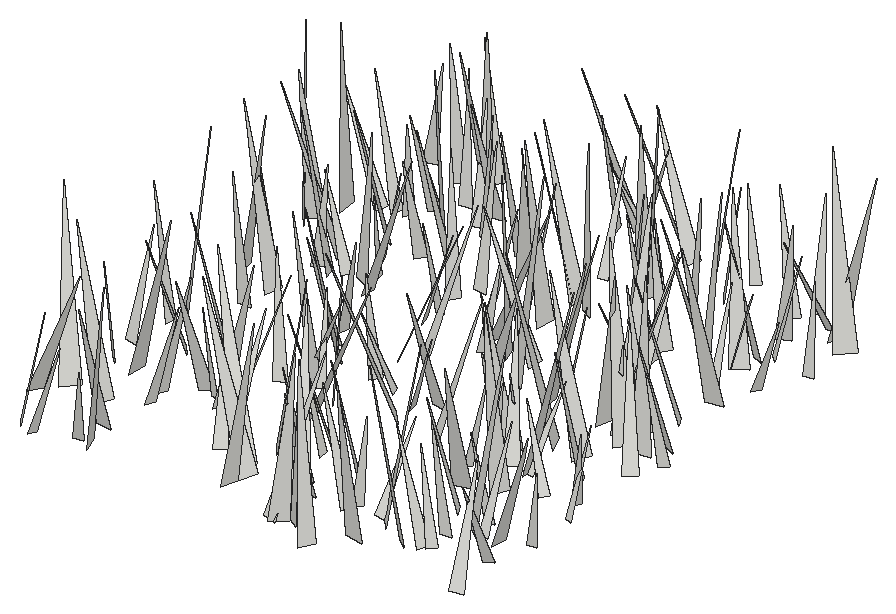
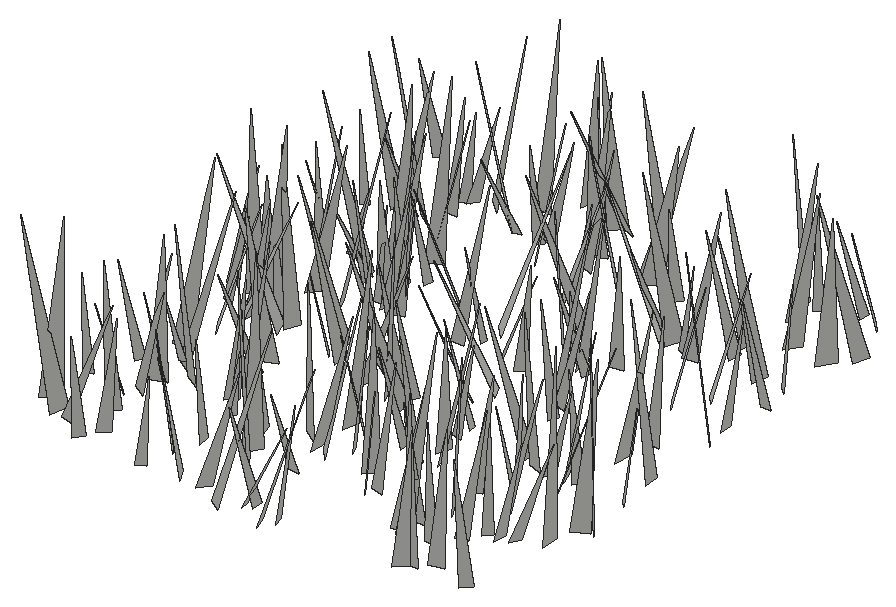
# SketchUp Ruby script. Lengths in inches.
U = 1.inch
M = Sketchup.active_model
def pt(a) = Geom::Point3d.new(a.map { |v| v * U })
def face(e, loops, mat)
  f = e.add_face(loops[0].map { |a| pt(a) })
  loops[1..].each { |l| e.add_face(l.map { |a| pt(a) }).erase! }
  f.material = f.back_material = mat if mat
  f
end
# faces: each face lists its corners as indices into pts; further lists are holes
def faces(e, pts, list, mat = nil) = list.each { |f| face(e, (f[0].is_a?(Array) ? f : [f]).map { |l| l.map { |i| pts[i] } }, mat) }
# xy, xz, yz: faces in a plane at the given z, y or x. An outline is a flat list of corners, or four numbers for a rectangle; further outlines are holes
def ring(l) = l.size == 4 ? [[l[0], l[1]], [l[2], l[1]], [l[2], l[3]], [l[0], l[3]]] : l.each_slice(2).to_a
def flat(e, list, mat, &to3) = list.each { |f| face(e, (f[0].is_a?(Array) ? f : [f]).map { |l| ring(l).map { |u, v| to3.(u, v) } }, mat) }
def xy(e, z, list, mat = nil) = flat(e, list, mat) { |x, y| [x, y, z] }
def xz(e, y, list, mat = nil) = flat(e, list, mat) { |x, z| [x, y, z] }
def yz(e, x, list, mat = nil) = flat(e, list, mat) { |y, z| [x, y, z] }
def lines(e, pts, list) = list.each { |a, b| e.add_line(pt(pts[a]), pt(pts[b])) }
# prism: a flat outline (further loops are holes) pulled along v
def prism(e, loops, v, mat = nil)
  f = face(e, loops, mat); d = Geom::Vector3d.new(v.map { |x| x * U })
  f.pushpull(f.normal.samedirection?(d) ? d.length : -d.length)
end
def box(e, o, s, mat = nil) = prism(e, [[o, [o[0] + s[0], o[1], o[2]], [o[0] + s[0], o[1] + s[1], o[2]], [o[0], o[1] + s[1], o[2]]]], [0, 0, s[2]], mat)
def at(x, y, z, deg = 0) = Geom::Transformation.translation(pt([x, y, z])) * Geom::Transformation.rotation(ORIGIN, Z_AXIS, deg.degrees)
def axes(o, x, y, z) = Geom::Transformation.new([*x, 0, *y, 0, *z, 0, *pt(o).to_a, 1])
def part(name) = M.definitions.add(name)
# library, detail: a bought-in or finely detailed component or shape, given as its bounding box
def library(name, o, s) = part(name).tap { |d| box(d.entities, o, s) }
def detail(e, o, s) = box(e.add_group.entities, o, s)
def put(e, d, t, mat = nil) = e.add_instance(d, t).tap { |i| i.material = mat if mat }
def group(e, t, mat = nil) = e.add_group.tap { |g| g.transformation = t; g.material = mat if mat }.entities
root = M.entities
c1 = part("fur_instance\#9")
p = [[0.8125,0,1.79],[0.67,-0.02,1.48],[0,-0.11,0],[0,0.11,0]]
faces(c1.entities,p,[[0,1,2,3]])
put(root,c1,axes([454.47,144.27,-21.66],[-5.7343,-4.84539,3.53032],[-5.45543,6.24306,-0.29262],[2.4858,2.5238,7.50162]))
put(root,c1,axes([456.54,114.57,-21.66],[-6.24341,4.5177,1.05822],[4.50521,6.32678,-0.4296],[1.11019,-0.26807,7.69449]))
put(root,c1,axes([456.32,126.54,-21.66],[-5.31115,0.249,1.00047],[0.14264,5.37711,-0.58108],[1.02108,0.54405,5.28514]))
put(root,c1,axes([455.14,139.93,-21.66],[-2.6203,-2.567,1.06702],[-2.53846,2.80716,0.51965],[1.13325,0.35259,3.63117]))
put(root,c1,axes([455.01,145.13,-21.66],[3.62749,-5.55241,1.8821],[-5.65778,-3.89547,-0.58748],[-1.5366,1.23544,6.60627]))
put(root,c1,axes([455.76,147.71,-21.66],[7.3985,0.06507,3.2704],[0.28828,-8.06925,-0.49163],[-3.25831,-0.56619,7.38244]))
put(root,c1,axes([457.83,149.07,-21.66],[-4.93751,1.50851,0.32737],[1.53378,4.91815,0.47027],[0.1741,-0.54591,5.14135]))
put(root,c1,axes([455.94,122.39,-21.66],[0.58745,4.61701,1.14714],[4.75417,-0.52722,-0.31264],[0.17496,-1.17604,4.64372]))
put(root,c1,axes([456.65,119.57,-21.66],[-2.76326,-3.0585,1.38467],[-3.15346,2.97986,0.28892],[1.15213,0.82059,4.11176]))
put(root,c1,axes([455.68,136.01,-21.66],[6.8953,0.9557,1.85973],[1.13553,-7.09282,-0.56526],[-1.75571,-0.83402,6.93822]))
put(root,c1,axes([456.08,128.73,-21.66],[5.70767,4.90783,2.44546],[5.23724,-5.92496,-0.33273],[-1.62433,-1.85811,7.52021]))
put(root,c1,axes([459,149.46,-21.66],[-5.26641,1.25593,0.32091],[1.22212,5.2582,-0.5227],[0.43216,0.43524,5.3888]))
put(root,c1,axes([456.43,156.58,-21.66],[2.66304,-4.00114,1.09323],[-4.14622,-2.60379,0.57024],[-0.11461,1.22768,4.77239]))
put(root,c1,axes([454.9375,112.5,-21.66],[5.86888,-2.59714,0.14419],[-2.59865,-5.83866,0.60558],[0.11385,0.61201,6.38922]))
put(root,c1,axes([459.375,134.63,-21.66],[-7.31689,1.04904,1.18508],[0.99417,7.40794,-0.41938],[1.23147,0.25252,7.3798]))
put(root,c1,axes([459.79,141.79,-21.66],[-6.57116,-2.81105,0.67584],[-2.85659,6.57143,-0.44162],[0.44572,0.67315,7.13352]))
put(root,c1,axes([457.24,107.96,-21.66],[3.19373,2.97376,0.94617],[2.91746,-3.32577,0.60507],[-1.10768,-0.18543,4.3217]))
put(root,c1,axes([459.01,131.72,-21.66],[-0.51846,-5.08764,2.15235],[-5.51728,0.36879,-0.45728],[-0.27624,2.18298,5.0935]))
put(root,c1,axes([459.97,114.18,-21.66],[-6.35948,3.06032,1.72749],[3.24757,6.48259,0.47123],[1.34279,-1.18457,7.04176]))
put(root,c1,axes([459.87,123.89,-21.66],[-3.79874,-3.55526,0.6962],[-3.51199,3.8615,0.55657],[0.88909,0.06302,5.17306]))
put(root,c1,axes([460.84,139.38,-21.66],[-6.09908,-2.25868,1.59557],[-2.41433,6.23322,-0.4051],[1.3485,0.94419,6.49124]))
put(root,c1,axes([459.98,155.57,-21.66],[1.65081,-5.08845,2.41171],[-5.51574,-1.96719,-0.37505],[-1.13372,2.16141,5.33637]))
put(root,c1,axes([458.8125,107.37,-21.66],[3.85375,-0.57416,0.66525],[-0.65849,-3.86826,0.47595],[-0.58191,0.57487,3.8671]))
put(root,c1,axes([459.56,139.55,-21.66],[2.82184,-3.33686,1.43593],[-3.57868,-2.86589,0.37288],[-0.62414,1.34588,4.35412]))
put(root,c1,axes([461.29,145.62,-21.66],[-3.14093,-4.54056,1.19879],[-4.68857,3.11384,-0.49041],[0.26658,1.26749,5.49924]))
put(root,c1,axes([461.63,126.26,-21.66],[-4.56615,-2.82263,0.99228],[-2.92894,4.58662,-0.43101],[0.61084,0.89289,5.35081]))
put(root,c1,axes([460.02,149.57,-21.66],[3.44775,-2.42349,1.09947],[-2.43313,-3.5995,-0.30427],[-1.07797,0.37336,4.2033]))
put(root,c1,axes([458.95,119.33,-21.66],[7.358,-0.55238,1.16955],[-0.51092,-7.44716,-0.30295],[-1.18825,-0.21839,7.37248]))
put(root,c1,axes([461.96,139.97,-21.66],[-3.54918,2.04608,0.76374],[2.14815,3.53344,0.51649],[0.39398,-0.83357,4.06404]))
put(root,c1,axes([461.09,151.22,-21.66],[1.69834,-4.62751,0.65795],[-4.61755,-1.76962,-0.52709],[-0.72459,0.43091,4.90106]))
put(root,c1,axes([462.0625,157.12,-21.66],[-4.31803,3.62073,2.04082],[3.93255,4.51165,0.31626],[1.34522,-1.56695,5.62628]))
put(root,c1,axes([461.58,156.62,-21.66],[-0.58668,-6.43534,2.37936],[-6.81319,0.82822,0.56013],[0.80964,2.30643,6.43771]))
put(root,c1,axes([462.41,153.14,-21.66],[-0.09344,5.23116,1.72248],[5.50098,0.0052,0.28262],[-0.26677,-1.725,5.22436]))
put(root,c1,axes([462.25,111.37,-21.66],[-0.34138,-6.1128,0.75859],[-6.1403,0.39794,0.44341],[0.48829,0.7305,6.10625]))
put(root,c1,axes([462.02,108.7,-21.66],[1.68223,-3.64936,0.16027],[-3.63941,-1.65928,0.41825],[0.31341,0.31999,3.9966]))
put(root,c1,axes([462.75,143.23,-21.66],[3.22488,1.438,0.95498],[1.40641,-3.36208,0.31327],[-1.00092,-0.09099,3.51704]))
put(root,c1,axes([462.42,117.88,-21.66],[4.97792,-1.2009,1.19397],[-1.36113,-5.04298,0.6026],[-1.0075,0.87956,5.08515]))
put(root,c1,axes([464.18,148.36,-21.66],[-5.53367,-3.1899,2.46645],[-3.58117,5.81278,-0.51687],[1.85312,1.70777,6.3663]))
put(root,c1,axes([463.13,108.73,-21.66],[6.28919,2.00514,2.27548],[2.25266,-6.59596,-0.4138],[-2.03074,-1.10685,6.58812]))
put(root,c1,axes([462.73,116.125,-21.66],[4.30722,-1.10997,0.82887],[-1.21703,-4.32511,0.53238],[-0.66174,0.72977,4.41597]))
put(root,c1,axes([463.48,139.78,-21.66],[-2.04646,-5.42862,2.85461],[-5.95901,2.47232,0.42963],[1.45222,2.49488,5.78561]))
put(root,c1,axes([464.09,141.01,-21.66],[-3.40135,-0.48301,1.73948],[-0.24917,3.80046,0.56808],[1.78802,-0.38922,3.38818]))
put(root,c1,axes([464.97,151.35,-21.66],[-0.50295,4.78104,0.71911],[4.81704,0.43358,0.48636],[-0.41423,-0.76294,4.78276]))
put(root,c1,axes([464.6,145.21,-21.66],[2.46831,-3.73303,1.12427],[-3.72872,-2.64901,-0.60947],[-1.13849,0.58247,4.43358]))
put(root,c1,axes([464.51,153.73,-21.66],[-1.5232,-7.73744,1.34983],[-7.81047,1.63722,0.57115],[0.82858,1.20901,7.86523]))
put(root,c1,axes([464.74,120.18,-21.66],[1.62052,-5.44249,0.65001],[-5.43307,-1.68456,-0.55967],[-0.72449,0.45919,5.65098]))
put(root,c1,axes([465.52,153.15,-21.66],[0.67121,-5.58126,0.90748],[-5.6399,-0.72653,-0.2969],[-0.40679,0.86382,5.61363]))
put(root,c1,axes([465.89,119.6875,-21.66],[-1.30466,-3.28465,1.2487],[-3.51229,1.2605,-0.354],[0.10971,1.29326,3.5165]))
put(root,c1,axes([466.34,150.25,-21.66],[2.39277,4.07076,1.54907],[4.21231,-2.6123,0.35825],[-1.10775,-1.14055,4.7083]))
put(root,c1,axes([464.87,138.76,-21.66],[6.15775,0.09619,0.89999],[0.03195,-6.20791,0.44493],[-0.90455,0.43558,6.14241]))
put(root,c1,axes([467.77,131.55,-21.66],[-1.24841,-4.57565,0.91997],[-4.66472,1.19209,-0.401],[-0.15278,0.99186,4.72592]))
put(root,c1,axes([468.14,124.5,-21.66],[-1.55203,4.86816,1.43833],[5.0761,1.479,0.47157],[-0.03172,-1.51332,5.08777]))
put(root,c1,axes([467.01,133.26,-21.66],[4.35751,-1.25814,0.68683],[-1.21703,-4.4086,-0.35441],[-0.75729,-0.15444,4.52164]))
put(root,c1,axes([469.375,143.32,-21.66],[-6.2182,-2.45212,1.53392],[-2.39925,6.40419,0.51167],[1.61537,0.0727,6.66461]))
put(root,c1,axes([467.15,119.01,-21.66],[6.16664,-2.56617,1.31423],[-2.70082,-6.22755,0.51287],[-1.00896,0.98602,6.65955]))
put(root,c1,axes([469.31,129.83,-21.66],[-3.91198,-5.41617,1.52932],[-5.50053,4.07361,0.35664],[1.19076,1.02376,6.67167]))
put(root,c1,axes([470.28,125.84,-21.66],[-6.61174,-0.50833,1.66504],[-0.62205,6.79727,-0.39495],[1.62598,0.53342,6.61948]))
put(root,c1,axes([469.25,117.98,-21.66],[-0.73079,4.32054,0.1844],[4.30671,0.74406,-0.36572],[0.39156,-0.12013,4.36662]))
put(root,c1,axes([470.26,141.9,-21.66],[-5.1029,2.41175,1.4356],[2.37658,5.2976,-0.4521],[1.4931,-0.1897,5.62599]))
put(root,c1,axes([470.33,149.57,-21.66],[-1.33118,-5.02308,1.66852],[-5.29255,1.28443,-0.35575],[0.06525,1.70478,5.18429]))
put(root,c1,axes([470.93,114.07,-21.66],[-3.67286,3.55796,0.5072],[3.52102,3.70767,-0.51167],[0.72023,0.01818,5.08794]))
put(root,c1,axes([470.8,139.6875,-21.66],[-0.62514,-3.66803,1.11265],[-3.82799,0.53943,-0.37244],[-0.19721,1.15663,3.70223]))
put(root,c1,axes([468.4,119.11,-21.66],[5.68273,3.19615,0.64935],[3.24559,-5.67036,-0.49352],[-0.32122,-0.74969,6.50117]))
put(root,c1,axes([471.07,150.01,-21.66],[-3.53133,-2.30027,1.49102],[-2.55807,3.63918,-0.44418],[0.98523,1.20406,4.19097]))
put(root,c1,axes([471.07,125.63,-21.66],[-0.33834,3.74046,0.53618],[3.75079,0.26714,0.50319],[-0.45836,-0.57497,3.72187]))
put(root,c1,axes([469.18,126.7,-21.66],[3.86855,-0.79855,0.19754],[-0.81455,-3.85123,0.38332],[-0.11496,0.41562,3.93147]))
put(root,c1,axes([471.12,143.99,-21.66],[0.82489,5.68831,1.342],[5.81529,-0.93413,0.38496],[-0.58339,-1.2684,5.73491]))
put(root,c1,axes([473.84,113.25,-21.66],[-6.13421,5.52562,0.24546],[5.52788,6.11218,0.5523],[-0.18784,-0.57446,8.23747]))
put(root,c1,axes([470.72,138,-21.66],[4.18181,1.0835,0.53294],[1.13424,-4.18373,-0.39425],[-0.41412,-0.51766,4.30187]))
put(root,c1,axes([474.02,158.5625,-21.66],[-6.24569,-2.79636,0.92417],[-2.76847,6.31368,0.39421],[1.00464,0.01396,6.83176]))
put(root,c1,axes([475.15,111.96,-21.66],[-7.32829,2.58062,0.59876],[2.60966,7.33524,0.32553],[0.45582,-0.50666,7.76257]))
put(root,c1,axes([473.16,157.49,-21.66],[-4.36965,-1.59831,1.51111],[-1.58231,4.61869,0.30967],[1.52785,0.21216,4.64247]))
put(root,c1,axes([473.3125,129.15,-21.66],[-3.08367,2.72536,1.78242],[3.08151,3.23588,0.38343],[1.05304,-1.48834,4.09751]))
put(root,c1,axes([472.31,147.73,-21.66],[4.37125,-4.19897,0.80164],[-4.19734,-4.43318,-0.33332],[-0.81017,0.31203,6.05212]))
put(root,c1,axes([472.9,124.66,-21.66],[4.36466,2.86173,1.95624],[3.18404,-4.55325,-0.44325],[-1.3705,-1.46462,5.20032]))
put(root,c1,axes([472.875,143.14,-21.66],[4.10361,0.18993,0.89205],[0.09258,-4.17709,0.46346],[-0.90734,0.43277,4.08178]))
put(root,c1,axes([473.67,134.6,-21.66],[2.91229,5.1803,0.24137],[5.15397,-2.92189,0.52374],[-0.57474,0.04729,5.91968]))
put(root,c1,axes([472.66,132.68,-21.66],[5.42276,2.60915,0.23648],[2.58182,-5.41452,0.53583],[-0.44475,0.3811,5.9939]))
put(root,c1,axes([475.55,128.5,-21.66],[-3.47043,-1.20582,0.35373],[-1.16309,3.47557,0.43669],[0.47575,-0.29913,3.64791]))
put(root,c1,axes([474.26,116.47,-21.66],[5.20843,4.28763,1.83578],[4.29945,-5.48037,0.60158],[-1.80791,-0.68076,6.71935]))
put(root,c1,axes([476.55,157.2,-21.66],[-3.57731,-0.93265,0.01118],[-0.92223,3.54345,0.51048],[0.1395,-0.49118,3.66148]))
put(root,c1,axes([475.42,145.83,-21.66],[3.95748,1.9361,2.48086],[2.44941,-4.39763,-0.47534],[-1.97573,-1.57388,4.37997]))
put(root,c1,axes([477.72,147.11,-21.66],[-6.93734,1.12272,0.61983],[1.08478,6.95591,-0.45824],[0.68406,0.3553,7.01265]))
put(root,c1,axes([476.79,147.61,-21.66],[-5.18557,-4.32883,1.54546],[-4.49087,5.26797,-0.31293],[0.97941,1.23577,6.74766]))
put(root,c1,axes([473.3,121.72,-21.66],[6.47298,0.85818,0.33872],[0.84258,-6.4766,0.30739],[-0.37587,0.26066,6.52238]))
put(root,c1,axes([475.15,144.68,-21.66],[3.56693,3.32971,1.1246],[3.34181,-3.70943,0.38354],[-1.08812,-0.47732,4.86445]))
put(root,c1,axes([474.68,110.42,-21.66],[6.67765,-1.57713,2.05629],[-1.75682,-6.93326,0.38749],[-1.90506,0.86558,6.85042]))
put(root,c1,axes([477.46,119,-21.66],[-4.41159,-3.54695,0.73212],[-3.61607,4.3782,-0.57829],[0.20221,0.91078,5.63104]))
put(root,c1,axes([478.08,125.5625,-21.66],[-5.65228,-5.31186,0.60473],[-5.29476,5.68375,0.43618],[0.73959,0.09466,7.74428]))
put(root,c1,axes([476.91,151,-21.66],[0.03105,4.61747,0.04613],[4.59439,-0.03553,0.46309],[-0.46341,-0.04278,4.59429]))
put(root,c1,axes([477.31,118,-21.66],[-3.67755,-0.2078,1.11626],[-0.0694,3.8179,0.48208],[1.13331,-0.4405,3.65173]))
put(root,c1,axes([475.76,156.63,-21.66],[4.29201,-0.29938,0.77765],[-0.39482,-4.32378,0.51456],[-0.73381,0.57535,4.27156]))
put(root,c1,axes([477.78,143.18,-21.66],[-7.15931,0.95304,2.49675],[1.12982,7.54938,0.35801],[2.42189,-0.70454,7.21359]))
put(root,c1,axes([478.25,158.48,-21.66],[-4.17901,-5.88434,0.7845],[-5.89024,4.22956,0.34775],[0.73891,0.43633,7.20893]))
put(root,c1,axes([476.8,137.21,-21.66],[3.29573,-2.04708,1.27302],[-2.29025,-3.33183,0.57152],[-0.75223,1.17531,3.83742]))
put(root,c1,axes([478.625,137.91,-21.66],[-6.27895,-2.5321,2.5957],[-2.9165,6.61067,-0.60625],[2.15482,1.56906,6.74309]))
put(root,c1,axes([479.55,112.49,-21.66],[-3.35316,6.39569,0.22234],[6.39729,3.34326,0.30873],[-0.17041,-0.34016,7.2148]))
put(root,c1,axes([478.91,114.51,-21.66],[-1.67954,-4.60165,1.09216],[-4.72861,1.65608,-0.29411],[0.09072,1.12742,4.88974]))
put(root,c1,axes([480.54,156.83,-21.66],[-5.38349,2.8617,0.60302],[2.91403,5.35589,0.59819],[0.24775,-0.81245,6.06741]))
put(root,c1,axes([479.19,146.21,-21.66],[3.04497,5.63186,2.55497],[5.93211,-3.46487,0.56775],[-1.7481,-1.94792,6.3771]))
put(root,c1,axes([476.43,138.89,-21.66],[6.73911,-0.51973,0.37006],[-0.5475,-6.72675,0.52311],[-0.32757,0.55072,6.73884]))
put(root,c1,axes([481.02,138.05,-21.66],[-6.42244,0.41118,0.57395],[0.45958,6.42194,0.54196],[0.53597,-0.57954,6.41273]))
put(root,c1,axes([478.06,127.52,-21.66],[3.62066,0.28745,0.41277],[0.34104,-3.60783,-0.479],[-0.36973,-0.51296,3.60033]))
put(root,c1,axes([479.46,128.8,-21.66],[-0.57876,-6.04691,0.53315],[-6.05695,0.61084,0.35302],[0.40347,0.49606,6.06428]))
put(root,c1,axes([478.83,136.14,-21.66],[3.52002,-2.83902,0.00242],[-2.82378,-3.50072,0.47096],[0.29379,0.3681,4.49764]))
put(root,c1,axes([480.15,108.1875,-21.66],[2.22729,6.28936,0.04999],[6.2767,-2.22605,0.40869],[-0.40191,0.08939,6.65956]))
put(root,c1,axes([480.11,112.73,-21.66],[0.60186,-6.09784,0.10298],[-6.0697,-0.58883,0.60707],[0.59415,0.16161,6.09732]))
put(root,c1,axes([480.29,152.07,-21.66],[6.26613,3.81902,2.82967],[4.24719,-6.60086,-0.4964],[-2.13385,-1.92357,7.3214]))
put(root,c1,axes([480.9,108.375,-21.66],[4.75602,-4.66812,2.75377],[-5.20371,-4.95731,0.58378],[-1.51526,2.37234,6.63855]))
put(root,c1,axes([481.125,150.5,-21.66],[6.49174,-3.69034,2.54193],[-3.75607,-6.92147,-0.45599],[-2.44375,0.83512,7.45341]))
put(root,c1,axes([481.98,108.71,-21.66],[3.06348,4.37723,2.06786],[4.6001,-3.39453,0.37061],[-1.50841,-1.46222,5.32989]))
put(root,c1,axes([481.62,135.09,-21.66],[4.31651,6.80061,2.35568],[7.01576,-4.58865,0.3914],[-1.60519,-1.76799,8.04533]))
put(root,c1,axes([482.56,115.86,-21.66],[-4.52954,-3.25843,1.35312],[-3.24257,4.71245,0.49358],[1.39071,0.3748,5.55792]))
put(root,c1,axes([483.625,112.92,-21.66],[-4.37438,2.14658,0.79892],[2.22863,4.38643,0.41683],[0.52851,-0.72986,4.85482]))
put(root,c1,axes([482.29,147.57,-21.66],[4.52412,1.43506,1.852],[1.32361,-4.8885,0.5546],[-1.93323,0.01133,4.71375]))
put(root,c1,axes([482.82,156.65,-21.66],[4.79862,3.05458,1.6678],[3.017,-5.06719,0.60002],[-1.73486,-0.36311,5.65661]))
put(root,c1,axes([482.41,124.64,-21.66],[3.35621,4.76804,0.53975],[4.75729,-3.3924,0.38655],[-0.62744,-0.21695,5.81798]))
put(root,c1,axes([484.83,106.73,-21.66],[-6.58758,2.43197,1.48528],[2.355,6.75255,-0.6115],[1.60454,0.07391,6.99549]))
put(root,c1,axes([485.49,147.43,-21.66],[-3.44021,1.49763,0.22694],[1.46636,3.43395,-0.43273],[0.37973,0.30751,3.72702]))
put(root,c1,axes([483.97,113.67,-21.66],[2.50338,-2.82714,1.30611],[-3.05988,-2.54469,0.35667],[-0.57944,1.22368,3.75931]))
put(root,c1,axes([484.77,151.61,-21.66],[4.11345,0.18865,1.81103],[0.00918,-4.47631,0.44541],[-1.8208,0.4036,4.09361]))
put(root,c1,axes([485.69,127.4,-21.66],[-3.35833,-3.2337,1.73378],[-3.57177,3.41915,-0.54142],[0.83981,1.61055,4.63056]))
put(root,c1,axes([485.76,146.98,-21.66],[-4.49863,-0.46507,1.40367],[-0.60193,4.68178,-0.37796],[1.35065,0.53749,4.50678]))
put(root,c1,axes([485.36,128.27,-21.66],[2.55514,-3.36467,0.69917],[-3.31318,-2.64324,-0.61213],[-0.91251,0.1757,4.18031]))
put(root,c1,axes([486.12,157.26,-21.66],[1.74245,-3.02379,2.07472],[-3.3962,-2.19711,-0.34987],[-1.38332,1.58534,3.47232]))
put(root,c1,axes([484.47,136.09,-21.66],[5.61379,-0.0924,1.25595],[-0.17391,-5.73971,0.3551],[-1.24727,0.38445,5.60331]))
put(root,c1,axes([486.77,127.85,-21.66],[-5.40914,1.11965,1.3835],[1.23539,5.5484,0.3398],[1.28121,-0.62292,5.51334]))
put(root,c1,axes([485.77,135.85,-21.66],[-2.4957,-1.61977,2.11338],[-2.18018,2.90599,-0.34732],[1.52869,1.50005,2.95492]))
put(root,c1,axes([485.67,154.14,-21.66],[3.79573,2.84609,1.46317],[3.05532,-3.89817,-0.34352],[-0.95191,-1.16307,4.73179]))
put(root,c1,axes([487.05,145.5,-21.66],[-4.02078,2.93374,1.78068],[3.22926,4.16274,0.43339],[1.1617,-1.41743,4.95839]))
put(root,c1,axes([486.23,113.38,-21.66],[-0.08905,4.06249,0.07241],[4.03019,0.09752,-0.5148],[0.51634,-0.06053,4.03072]))
put(root,c1,axes([487.45,143.49,-21.66],[5.36084,-0.19835,3.29768],[0.06393,-6.27827,-0.48156],[-3.30302,-0.44345,5.34285]))
put(root,c1,axes([485.42,134.33,-21.66],[6.99973,1.86447,1.44835],[1.77883,-7.14461,0.6004],[-1.55233,0.22015,7.21886]))
put(root,c1,axes([486.81,109.66,-21.66],[-0.69172,-7.26259,1.83893],[-7.46362,0.82804,0.46276],[0.64909,1.78171,7.28077]))
put(root,c1,axes([486.66,123.19,-21.66],[3.38987,-1.12165,1.00676],[-1.27426,-3.45624,0.43994],[-0.80492,0.7478,3.54341]))
put(root,c1,axes([488.33,124.95,-21.66],[5.38161,2.47127,3.67462],[2.66712,-6.4254,0.41515],[-3.53503,-1.08568,5.90733]))
put(root,c1,axes([487.21,112.875,-21.66],[5.30824,4.83924,1.79848],[4.88732,-5.54151,0.48577],[-1.6634,-0.83881,7.16657]))
put(root,c1,axes([489.05,125.22,-21.66],[-1.93628,5.55,0.46539],[5.55779,1.89356,0.54185],[-0.36056,-0.61659,5.85304]))
put(root,c1,axes([487.84,127.625,-21.66],[-0.65259,-3.58567,0.77528],[-3.62638,0.74954,0.41412],[0.55447,0.682,3.62097]))
put(root,c1,axes([489.5,129.76,-21.66],[-7.3935,-3.44968,1.78048],[-3.41196,7.60131,0.55924],[1.85173,0.23234,8.13949]))
put(root,c1,axes([488.4,139.61,-21.66],[-2.23719,7.0676,1.63885],[7.20712,2.3619,-0.34736],[0.83319,-1.45336,7.40509]))
put(root,c1,axes([488.31,141.06,-21.66],[-0.0626,5.05917,0.30688],[5.04763,0.09003,-0.45456],[0.45914,-0.29998,5.03909]))
put(root,c1,axes([488.04,124.28,-21.66],[2.26375,-3.28304,0.92587],[-3.40814,-2.22313,0.4499],[-0.14199,1.01955,3.96238]))
put(root,c1,axes([489.95,111.36,-21.66],[4.02018,4.80904,4.066],[5.52928,-5.00439,0.45193],[-3.01434,-2.76593,6.25176]))
put(root,c1,axes([488.11,120.59,-21.66],[2.21636,-6.61774,0.25451],[-6.61771,-2.20273,0.35418],[0.25535,0.35358,6.97003]))
put(root,c1,axes([490.18,117.72,-21.66],[-4.23671,-2.59002,0.97553],[-2.55905,4.34534,0.42292],[1.0541,0.13924,4.94763]))
put(root,c1,axes([491.55,111.82,-21.66],[-4.44101,1.77663,0.66677],[1.83519,4.45274,0.3588],[0.48276,-0.58331,4.76973]))
put(root,c1,axes([490.84,121.59,-21.66],[-6.55699,2.55506,2.62376],[2.8465,6.94107,0.35432],[2.30431,-1.30376,7.02829]))
put(root,c1,axes([492.32,129.3,-21.66],[-6.29408,3.56033,1.19684],[3.6784,6.31519,0.55815],[0.76008,-1.07993,7.20971]))
put(root,c1,axes([491.29,155.04,-21.66],[-3.65531,3.57205,1.42816],[3.77376,3.712,0.37448],[0.74692,-1.27356,5.09712]))
put(root,c1,axes([491.04,145.1875,-21.66],[3.25616,5.95918,2.11371],[6.15078,-3.5363,0.49462],[-1.46542,-1.60155,6.77272]))
put(root,c1,axes([490.75,125.05,-21.66],[0.42201,3.83383,0.13948],[3.79822,-0.3978,-0.55775],[0.53966,-0.19825,3.81644]))
put(root,c1,axes([491.75,114.22,-21.66],[0.28904,-4.61969,1.68996],[-4.89331,-0.44312,-0.3744],[-0.50298,1.65624,4.61355]))
put(root,c1,axes([492.09,112.18,-21.66],[-2.34318,3.21724,1.23905],[3.43189,2.31946,0.46753],[0.3286,-1.2829,3.95253]))
put(root,c1,axes([490.32,134.38,-21.66],[6.63287,-1.89646,1.66739],[-1.83678,-6.83922,-0.47211],[-1.73291,-0.0097,6.88248]))
put(root,c1,axes([492.88,143.76,-21.66],[-3.74984,-6.28849,1.24601],[-6.40364,3.74219,-0.38514],[0.30173,1.26879,7.3115]))
put(root,c1,axes([493.66,136.44,-21.66],[-3.87501,-4.05549,0.17386],[-4.05477,3.85598,-0.42797],[-0.18982,0.42113,5.59281]))
put(root,c1,axes([490.58,125.22,-21.66],[7.58691,1.58366,1.76713],[1.48707,-7.78642,0.59349],[-1.84915,0.23586,7.72768]))
put(root,c1,axes([492.99,146.72,-21.66],[-2.95923,6.17255,1.7602],[6.41346,2.92118,0.53848],[0.25723,-1.82266,6.82403]))
put(root,c1,axes([492.26,156.75,-21.66],[-3.32764,3.062,1.30373],[3.08153,3.53122,-0.42827],[1.25687,-0.55083,4.50173]))
put(root,c1,axes([493.12,148.69,-21.66],[-2.87551,-4.98025,1.4124],[-5.17006,2.84441,-0.49611],[0.26119,1.47404,5.72934]))
put(root,c1,axes([493.68,135.05,-21.66],[-5.54027,1.19429,0.93196],[1.15956,5.61711,-0.30487],[0.97482,0.10593,5.65933]))
put(root,c1,axes([493.75,123.18,-21.66],[-2.71204,2.5664,0.21286],[2.56651,2.66825,0.52947],[-0.21147,-0.53003,3.69611]))
put(root,c1,axes([493.58,132.7,-21.66],[-6.05615,5.17907,2.30301],[5.46239,6.23254,0.34836],[1.51293,-1.77094,7.96105]))
put(root,c1,axes([492.16,133.54,-21.66],[2.05705,-3.40779,1.21765],[-3.60141,-2.06493,0.30505],[-0.3543,1.20424,3.9688]))
put(root,c1,axes([493.17,117.51,-21.66],[-0.82021,3.34867,1.94688],[3.86928,0.61559,0.57127],[-0.18046,-2.02092,3.4]))
put(root,c1,axes([494.51,137.97,-21.66],[-5.00716,-3.11226,0.75462],[-3.18598,4.98296,-0.58898],[0.32424,0.90067,5.86608]))
put(root,c1,axes([493.23,143.45,-21.66],[0.25291,3.93977,0.05992],[3.89833,-0.25892,0.57035],[-0.57304,-0.02262,3.90646]))
put(root,c1,axes([490.86,135.11,-21.66],[6.96857,2.87265,0.80723],[2.85827,-7.01507,0.2896],[-0.85676,-0.03815,7.53188]))
put(root,c1,axes([492.21,146.86,-21.66],[3.27913,1.40298,0.59687],[1.4938,-3.23974,-0.59158],[-0.30522,-0.78299,3.51725]))
put(root,c1,axes([492.73,152.16,-21.66],[3.51068,-4.45404,1.06123],[-4.56743,-3.50052,0.41776],[-0.32136,1.09429,5.65587]))
put(root,c1,axes([492.92,115.91,-21.66],[4.37398,5.97616,2.1686],[6.29129,-4.44766,-0.43255],[-0.91492,-2.01317,7.39318]))
put(root,c1,axes([494.59,155.32,-21.66],[-0.95692,-4.60949,0.0097],[-4.59629,0.95343,-0.35816],[-0.34872,0.08227,4.69412]))
put(root,c1,axes([493.97,115.82,-21.66],[0.66695,4.37993,0.08385],[4.36286,-0.67176,0.3871],[-0.39533,-0.02429,4.41347]))
put(root,c1,axes([494.55,126.53,-21.66],[4.53456,1.85789,3.16607],[2.55783,-5.20835,-0.60709],[-2.63311,-1.85992,4.86266]))
put(root,c1,axes([493.96,149.53,-21.66],[2.60004,3.22909,0.64132],[3.22546,-2.66223,0.32783],[-0.65933,-0.2899,4.13277]))
put(root,c1,axes([494.83,141.57,-21.66],[0.47812,-7.3143,1.47747],[-7.45136,-0.54714,-0.29732],[-0.39895,1.45332,7.32388]))
put(root,c1,axes([496.67,129.51,-21.66],[-4.29612,3.71614,0.38084],[3.69784,4.31285,-0.36964],[0.52979,0.03157,5.66831]))
put(root,c1,axes([495.29,132.4,-21.66],[1.282,-6.99581,3.06835],[-7.6361,-1.26107,0.31524],[-0.21483,3.07701,7.10532]))
put(root,c1,axes([496.43,134.28,-21.66],[-1.84979,-4.95748,0.73449],[-4.97918,1.90688,0.3307],[0.56907,0.57009,5.281]))
put(root,c1,axes([497.51,153.36,-21.66],[-5.36752,5.77658,2.45123],[6.12108,5.53013,0.37117],[1.38195,-2.05828,7.87664]))
put(root,c1,axes([496.625,113.09,-21.66],[1.2889,-4.23263,0.01136],[-4.22076,-1.28617,-0.32791],[-0.31699,-0.08469,4.41236]))
put(root,c1,axes([496.32,123.68,-21.66],[3.38817,-1.89067,0.4047],[-1.85762,-3.4096,-0.37677],[-0.53632,-0.13453,3.86165]))
put(root,c1,axes([495.9375,145.02,-21.66],[3.40491,-1.73217,0.1961],[-1.74293,-3.39081,0.31125],[-0.03288,0.3664,3.80749]))
put(root,c1,axes([497.3,121.51,-21.66],[1.47589,3.3854,0.35503],[3.34161,-1.51469,0.55196],[-0.64858,-0.1002,3.65165]))
put(root,c1,axes([497.7,132.04,-21.66],[1.52237,-3.55739,1.37163],[-3.65271,-1.78416,-0.57315],[-1.09275,1.00785,3.82677]))
put(root,c1,axes([497.6,108.13,-21.66],[-1.60174,4.9541,0.61833],[4.97114,1.64265,-0.28364],[0.46172,-0.4996,5.19887]))
put(root,c1,axes([495.43,115.76,-21.66],[5.75538,-1.33671,0.29214],[-1.31847,-5.75568,-0.36093],[-0.36579,-0.28603,5.89753]))
put(root,c1,axes([495.8,154.6,-21.66],[7.40162,-2.04644,1.37858],[-2.14984,-7.48787,0.42713],[-1.21103,0.78507,7.66743]))
put(root,c1,axes([497.63,148.94,-21.66],[0.95056,-3.70171,1.6828],[-4.06505,-0.90725,0.30052],[-0.09921,1.70654,3.80998]))
put(root,c1,axes([497.57,116.89,-21.66],[0.85171,-3.4207,0.8533],[-3.50883,-0.73716,0.54719],[0.34265,0.95401,3.48241]))
